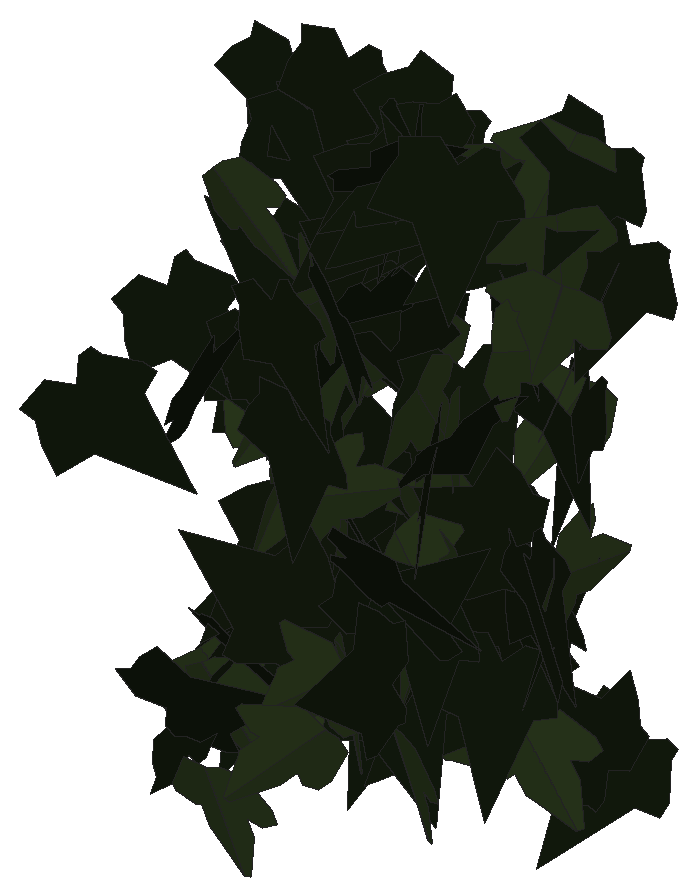
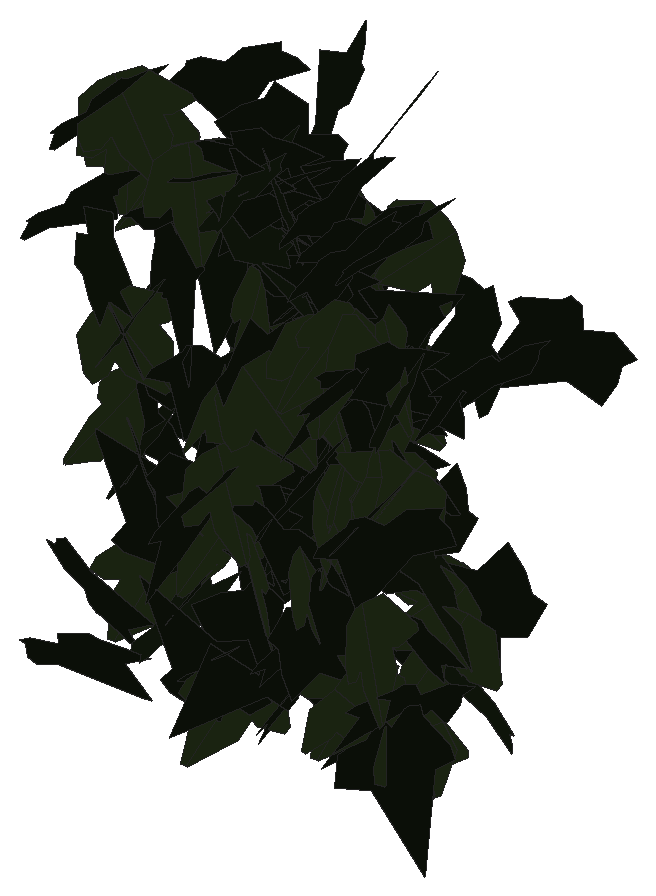
# SketchUp Ruby script. Lengths in inches.
U = 1.inch
M = Sketchup.active_model
def pt(a) = Geom::Point3d.new(a.map { |v| v * U })
def face(e, loops, mat)
  f = e.add_face(loops[0].map { |a| pt(a) })
  loops[1..].each { |l| e.add_face(l.map { |a| pt(a) }).erase! }
  f.material = f.back_material = mat if mat
  f
end
# faces: each face lists its corners as indices into pts; further lists are holes
def faces(e, pts, list, mat = nil) = list.each { |f| face(e, (f[0].is_a?(Array) ? f : [f]).map { |l| l.map { |i| pts[i] } }, mat) }
# xy, xz, yz: faces in a plane at the given z, y or x. An outline is a flat list of corners, or four numbers for a rectangle; further outlines are holes
def ring(l) = l.size == 4 ? [[l[0], l[1]], [l[2], l[1]], [l[2], l[3]], [l[0], l[3]]] : l.each_slice(2).to_a
def flat(e, list, mat, &to3) = list.each { |f| face(e, (f[0].is_a?(Array) ? f : [f]).map { |l| ring(l).map { |u, v| to3.(u, v) } }, mat) }
def xy(e, z, list, mat = nil) = flat(e, list, mat) { |x, y| [x, y, z] }
def xz(e, y, list, mat = nil) = flat(e, list, mat) { |x, z| [x, y, z] }
def yz(e, x, list, mat = nil) = flat(e, list, mat) { |y, z| [x, y, z] }
def lines(e, pts, list) = list.each { |a, b| e.add_line(pt(pts[a]), pt(pts[b])) }
# prism: a flat outline (further loops are holes) pulled along v
def prism(e, loops, v, mat = nil)
  f = face(e, loops, mat); d = Geom::Vector3d.new(v.map { |x| x * U })
  f.pushpull(f.normal.samedirection?(d) ? d.length : -d.length)
end
def box(e, o, s, mat = nil) = prism(e, [[o, [o[0] + s[0], o[1], o[2]], [o[0] + s[0], o[1] + s[1], o[2]], [o[0], o[1] + s[1], o[2]]]], [0, 0, s[2]], mat)
def at(x, y, z, deg = 0) = Geom::Transformation.translation(pt([x, y, z])) * Geom::Transformation.rotation(ORIGIN, Z_AXIS, deg.degrees)
def axes(o, x, y, z) = Geom::Transformation.new([*x, 0, *y, 0, *z, 0, *pt(o).to_a, 1])
def part(name) = M.definitions.add(name)
# library, detail: a bought-in or finely detailed component or shape, given as its bounding box
def library(name, o, s) = part(name).tap { |d| box(d.entities, o, s) }
def detail(e, o, s) = box(e.add_group.entities, o, s)
def put(e, d, t, mat = nil) = e.add_instance(d, t).tap { |i| i.material = mat if mat }
def group(e, t, mat = nil) = e.add_group.tap { |g| g.transformation = t; g.material = mat if mat }.entities
root = M.entities
M.materials.add("efeu1").color = [18, 25, 13]
M.materials.add("efeu2").color = [43, 57, 29]
c1 = part("ivyleaf_9")
p = [[1.54,2.16,1.25],[1.36,2.04,1.19],[-0.21,0.99,0.68],[-0.71,1.11,0.82],[-0.85,0.86,0.67],[-0.8,0.17,0.21],
  [-0.9,-0.01,0.1],[-0.67,-0.16,-0.02],[-0.08,-0.08,-0.05],[-0.03,-0.6,-0.4],[0.65,-0.88,-0.66],[0.83,-0.6,-0.49],
  [1.29,-0.42,-0.43],[1.8125,-0.07,-0.26],[1.21,0.44,0.15]]
faces(c1.entities,p,[[0,1,2,3,4,5,6,7,8,9,10,11,12,13,14]],"efeu1")
c2 = part("ivyleaf_10")
p = [[0,0.5,-0.03],[-0.0625,2.02,-0.43],[-0.19,2.01,-0.46],[-0.54,1.05,-0.29],[-0.52,0.625,-0.18],[-0.83,0.76,-0.28],
  [-1.16,0.64,-0.33],[-1.15,0.33,-0.24],[-0.77,-0.39,0.02],[-0.3,-0.51,0.16],[0.04,-0.48,0.23],[-0.02,2.01,-0.4375],
  [-0.06,2.01,-0.43],[0.04,-0.49,0.23],[0.67,-0.49,0.14],[1.38,0.36,-0.2],[1.375,0.51,-0.24],[0.81,0.65,-0.19],
  [0.62,0.59,-0.15],[0.6,1.09,-0.28],[0.5,1.23,-0.31]]
faces(c2.entities,p,[[0,1,2,3,4,5,6,7,8,9,10],[11,12,0,13,14,15,16,17,18,19,20]],"efeu2")
put(root,c1,axes([40.44,220.27,246.32],[0.16208,-0.38945,-0.26844],[0.03169,0.29207,-0.40459],[0.47194,0.11413,0.11936]))
put(root,c1,axes([40.98,221.25,242.32],[0.24181,0.19002,-0.39423],[-0.33477,-0.2098,-0.30646],[-0.28188,0.41216,0.02577]))
put(root,c1,axes([40.58,218.75,245.98],[-0.00232,-0.12946,-0.48294],[0.26446,0.40955,-0.11106],[0.42433,-0.25595,0.06657]))
put(root,c1,axes([40.75,221.67,244.9375],[-0.10521,-0.42408,-0.24307],[0.05609,0.23652,-0.43693],[0.48558,-0.11921,-0.0022]))
put(root,c1,axes([40.8,221.68,248.16],[-0.11399,-0.45265,0.17921],[0.02401,-0.18906,-0.46226],[0.48624,-0.09678,0.06484]))
put(root,c2,axes([40.99,220.93,242.1],[-0.09961,-0.48126,-0.09199],[0.00586,0.0927,-0.4913],[0.48994,-0.09896,-0.01282]))
put(root,c2,axes([41.04,221.55,243.63],[0.0308,-0.49854,-0.02258],[-0.00171,0.02252,-0.49949],[0.49905,0.03084,-0.00032]))
put(root,c1,axes([40.76,221.13,242.76],[0.14566,-0.34746,-0.32872],[0.08394,0.35686,-0.34001],[0.47089,0.04386,0.16229]))
put(root,c1,axes([41.27,219.52,242],[-0.37845,0.28286,-0.16361],[-0.1307,0.09841,0.47247],[0.29949,0.40038,-0.00055]))
put(root,c1,axes([40.91,221.3125,246.08],[0.02171,-0.27187,0.41907],[0.0689,-0.41382,-0.27204],[0.49475,0.06956,0.01949]))
put(root,c2,axes([41.41,220.84,246.49],[-0.27204,0.09807,0.40789],[-0.391,0.1169,-0.28889],[-0.15202,-0.47615,0.01309]))
put(root,c1,axes([41.27,221.42,246.47],[-0.33694,-0.35984,0.08358],[-0.06432,-0.05425,-0.49287],[0.36378,-0.34289,-0.00974]))
put(root,c2,axes([41.23,221.18,245.18],[0.04777,0.23287,-0.43987],[-0.10845,-0.42641,-0.23752],[-0.48575,0.1181,0.00977]))
put(root,c2,axes([40.98,221.0625,245.12],[0.36958,0.19046,0.27772],[0.22443,0.16812,-0.41396],[-0.25107,0.43065,0.03878]))
put(root,c1,axes([41,221.375,245.02],[0.26014,-0.39878,-0.15267],[-0.02205,0.16598,-0.47113],[0.42643,0.25185,0.06877]))
put(root,c2,axes([40.95,220.84,242.18],[-0.27106,-0.09475,-0.40933],[0.42005,-0.05039,-0.2665],[0.00925,-0.48835,0.10692]))
put(root,c2,axes([41.0625,220.44,247.59],[-0.34913,0.11494,-0.33897],[0.32423,-0.099,-0.36752],[-0.1516,-0.47643,-0.0054]))
put(root,c2,axes([41.33,221.57,242.76],[0.1825,0.34529,-0.3122],[-0.14436,-0.27682,-0.39055],[-0.44256,0.23268,-0.00135]))
put(root,c1,axes([41.35,219.25,245.77],[0.08753,0.14877,0.46926],[0.128,0.45335,-0.1676],[-0.47535,0.14947,0.04128]))
put(root,c1,axes([41.22,221.6875,247.97],[0.05816,-0.48707,-0.09686],[-0.01172,0.09615,-0.49053],[0.49647,0.05933,-0.00023]))
put(root,c2,axes([41.27,219.92,242.76],[-0.33136,-0.26762,-0.26188],[0.24862,0.10423,-0.4211],[0.27999,-0.40928,0.06399]))
put(root,c2,axes([41.3,221.33,242.82],[-0.38739,-0.23581,-0.21053],[0.23575,0.00633,-0.44089],[0.2106,-0.44086,0.10628]))
put(root,c1,axes([41.27,221.31,248.05],[-0.04877,-0.4417,-0.22918],[0.0279,0.22749,-0.44438],[0.49683,-0.05613,0.00246]))
put(root,c1,axes([41.8,220.65,246.45],[-0.00609,0.13398,0.48168],[-0.47214,0.15693,-0.04962],[-0.16447,-0.45544,0.1246]))
put(root,c1,axes([41.27,221.42,246.4],[0.19819,-0.38355,-0.25221],[-0.01826,0.26791,-0.42177],[0.45868,0.1764,0.09218]))
put(root,c1,axes([41.3125,220.55,246.05],[-0.18136,-0.21796,-0.41183],[0.33478,0.24642,-0.27785],[0.32409,-0.37652,0.05655]))
put(root,c1,axes([41.66,221.69,243.68],[-0.13173,0.22415,-0.42709],[0.17406,-0.39081,-0.25879],[-0.44984,-0.21686,0.02493]))
put(root,c1,axes([41.45,221.67,248.51],[0.00727,-0.49889,0.03256],[-0.01592,-0.03278,-0.49867],[0.49969,0.00622,-0.01636]))
put(root,c1,axes([41.89,219.7,243.48],[-0.25759,0.413,0.11435],[-0.07536,0.08768,-0.48645],[-0.42186,-0.26784,0.01707]))
put(root,c1,axes([41.22,219.3,242.54],[0.10449,-0.13173,0.47088],[0.45638,-0.14656,-0.14227],[0.1755,0.45953,0.08961]))
put(root,c1,axes([41.68,220.38,242.96],[-0.45556,-0.12577,-0.16324],[0.15565,0.04957,-0.47256],[0.13505,-0.48138,-0.00601]))
put(root,c2,axes([41.69,221.48,246.7],[-0.34193,-0.364,-0.02433],[0.01532,0.01898,-0.4994],[0.36449,-0.34226,-0.00183]))
put(root,c2,axes([41.59,221.29,246.75],[-0.09639,-0.32118,-0.37088],[0.19044,0.32384,-0.32994],[0.45215,-0.20487,0.0599]))
put(root,c2,axes([41.64,221.45,244.79],[0.12284,-0.42404,0.23474],[0.11413,-0.21004,-0.43915],[0.47105,0.16147,0.0452]))
put(root,c2,axes([41.78,221.57,244.06],[0.07186,-0.49282,0.04434],[-0.00324,-0.04528,-0.49794],[0.4948,0.07128,-0.0097]))
put(root,c2,axes([41.75,221.02,244.75],[0.10985,-0.41658,-0.25376],[0.05967,0.26964,-0.41681],[0.48412,0.06129,0.10896]))
put(root,c2,axes([41.64,219.52,242.85],[-0.41948,0.06518,-0.26417],[0.25554,-0.07237,-0.42363],[-0.09346,-0.49042,0.0274]))
put(root,c1,axes([41.52,220.88,245.39],[-0.13979,-0.11186,-0.46685],[0.44368,0.15558,-0.17013],[0.18333,-0.46182,0.05576]))
put(root,c1,axes([42.12,221.375,247.29],[-0.44983,-0.21695,0.02423],[-0.0134,-0.02796,-0.49904],[0.21789,-0.44961,0.01934]))
put(root,c2,axes([42.15,220.9,245.96],[-0.12388,-0.47377,0.10097],[0.00241,-0.10482,-0.48888],[0.4844,-0.12064,0.02825]))
put(root,c1,axes([41.92,221.36,243.24],[0.1556,-0.42092,-0.22049],[-0.02761,0.22361,-0.44636],[0.47437,0.15109,0.04634]))
put(root,c2,axes([42.34,221.72,246.01],[-0.26973,-0.3071,0.28798],[-0.19102,-0.21551,-0.40874],[0.37517,-0.33052,-0.00107]))
put(root,c1,axes([42.32,219.89,244.6],[-0.48355,-0.12698,-0.00729],[0.00658,0.00363,-0.49994],[0.12702,-0.48359,-0.00184]))
put(root,c2,axes([42.46,219.96,247.04],[-0.2431,0.12036,0.42002],[-0.40345,0.12267,-0.26867],[-0.16772,-0.46954,0.03748]))
put(root,c1,axes([42.04,221.65,244.44],[-0.29825,-0.19991,-0.34797],[0.3432,0.09763,-0.35026],[0.20799,-0.44778,0.07898]))
put(root,c1,axes([42.16,221.46,244.66],[-0.0575,-0.3964,0.29926],[-0.00934,-0.30034,-0.39963],[0.4966,-0.05155,0.02713]))
put(root,c1,axes([41.91,219.43,243.29],[0.1469,-0.27619,0.39005],[0.32512,-0.24135,-0.29334],[0.35031,0.33981,0.10868]))
put(root,c1,axes([42.26,221.01,246.83],[-0.18566,-0.31143,0.3443],[-0.02327,-0.3641,-0.34189],[0.46367,-0.14298,0.1207]))
put(root,c2,axes([42.33,218.61,242.38],[-0.49475,0.0394,-0.06056],[0.06045,-0.00383,-0.49632],[-0.03957,-0.49843,-0.00098]))
put(root,c2,axes([42.3,219.82,245.26],[-0.012,0.27146,-0.41972],[-0.01434,-0.41986,-0.27113],[-0.49965,0.00553,0.01786]))
put(root,c1,axes([42.15,221.16,242.53],[0.21146,-0.44611,-0.07917],[-0.02916,0.07379,-0.49367],[0.45214,0.2134,0.00519]))
put(root,c1,axes([42.625,220.99,247.81],[-0.3012,-0.33508,0.2168],[-0.15926,-0.14814,-0.45021],[0.36595,-0.34026,-0.01749]))
put(root,c1,axes([42.64,220.5,246.95],[-0.11834,0.39291,-0.28568],[0.07911,-0.27452,-0.41034],[-0.47931,-0.14232,0.00281]))
put(root,c1,axes([42.56,221.63,245.84],[-0.00384,-0.03793,0.49854],[-0.27489,-0.41629,-0.03379],[0.41764,-0.27435,-0.01766]))
put(root,c1,axes([42.41,221.37,248.26],[-0.26418,-0.00086,-0.42451],[0.41127,-0.12443,-0.25569],[-0.1052,-0.48427,0.06645]))
put(root,c1,axes([42.87,221.25,247.58],[-0.32351,0.38102,0.01303],[-0.06502,-0.03831,-0.49427],[-0.37566,-0.32149,0.07433]))
put(root,c1,axes([42.64,220.98,242.76],[-0.43786,-0.13681,-0.19891],[0.19256,0.05055,-0.45866],[0.14561,-0.47825,0.00842]))
put(root,c2,axes([42.64,220.36,243.51],[-0.34181,0.35785,0.0715],[-0.04332,0.05749,-0.49479],[-0.36234,-0.34444,-0.0083]))
put(root,c1,axes([42.77,221.49,248.53],[-0.44501,-0.22653,0.02555],[-0.01944,-0.01812,-0.49929],[0.22713,-0.44537,0.00732]))
put(root,c1,axes([42.43,221.36,242.98],[0.46637,0.17209,0.05369],[0.04903,0.0222,-0.49709],[-0.17347,0.46893,0.00383]))
put(root,c1,axes([42.67,220.87,243.65],[0.27045,-0.40309,0.1199],[-0.04156,0.11624,0.48452],[-0.41848,-0.27205,0.02937]))
put(root,c1,axes([42.79,221.3,247.87],[-0.33715,-0.29243,0.22543],[-0.05136,-0.26516,-0.42078],[0.36564,-0.30688,0.14876]))
put(root,c1,axes([42.64,220.6,248.29],[0.3319,0.3619,0.09417],[0.05805,0.07452,-0.491],[-0.36942,0.33686,0.00745]))
put(root,c1,axes([43.12,218.76,244.36],[-0.10997,0.17206,0.4564],[-0.45229,0.13917,-0.16144],[-0.18259,-0.44836,0.12503]))
put(root,c2,axes([42.88,221.15,243.65],[0.28172,-0.32908,-0.24968],[-0.15301,0.19758,-0.43307],[0.38369,0.32042,0.01062]))
put(root,c2,axes([42.61,219.82,245.11],[-0.07786,-0.08843,-0.48592],[0.27228,0.40273,-0.11692],[0.41207,-0.28282,-0.01456]))
put(root,c1,axes([42.57,221.66,248.11],[-0.00778,-0.38645,0.31717],[0.14645,-0.30505,-0.3681],[0.47801,0.08717,0.11793]))
put(root,c1,axes([43.09,221.23,248.28],[-0.47415,-0.08477,0.13414],[-0.10575,-0.1463,-0.46627],[0.1183,-0.47054,0.12081]))
put(root,c1,axes([42.67,219.43,246.02],[0.03892,-0.47276,0.15805],[0.02159,-0.15679,-0.47429],[0.49802,0.04374,0.00821]))
put(root,c1,axes([43.25,220.92,243.8125],[-0.34996,-0.03313,0.35557],[-0.35478,-0.02453,-0.35147],[0.04073,-0.4983,-0.00633]))
put(root,c1,axes([43.25,219.9,243.76],[-0.1896,0.01229,0.4625],[-0.45465,-0.09757,-0.18378],[0.08574,-0.49023,0.04817]))
put(root,c1,axes([43.25,219.85,243.17],[-0.00908,0.00988,0.49982],[-0.40507,0.29283,-0.01314],[-0.29298,-0.40516,0.00269]))
put(root,c1,axes([43.15,221.28,248.12],[-0.49084,-0.09467,-0.01088],[0.0104,0.00351,-0.49988],[0.09472,-0.49094,-0.00147]))
put(root,c2,axes([43.06,221.36,244.65],[-0.21097,-0.4433,0.09475],[-0.02826,-0.09144,-0.49075],[0.45243,-0.21242,0.01352]))
put(root,c2,axes([42.87,221.3125,242.27],[-0.26277,-0.32913,-0.26949],[0.2271,0.15929,-0.41599],[0.35969,-0.34103,0.06578]))
put(root,c1,axes([43.04,221.45,242.47],[-0.31424,-0.33366,0.19981],[-0.04742,-0.2221,-0.44545],[0.38601,-0.29891,0.10795]))
put(root,c1,axes([42.85,218.82,247.64],[0.2356,-0.43759,-0.05489],[-0.0199,0.05161,-0.49693],[0.44056,0.23634,0.0069]))
put(root,c1,axes([42.92,221.56,242.23],[-0.1764,0.1063,0.45561],[0.39368,-0.22936,0.20593],[0.25278,0.43139,-0.00278]))
put(root,c2,axes([43.28,221.6,248.16],[-0.2544,-0.42934,0.03079],[-0.01309,-0.02803,-0.49904],[0.43024,-0.25472,0.00302]))
put(root,c2,axes([43.2,221.27,245.52],[-0.06899,0.44621,-0.21478],[0.01086,-0.21544,-0.45107],[-0.4951,-0.06691,0.02004]))
put(root,c1,axes([43.125,221.59,244.43],[0.15993,-0.38066,-0.28199],[-0.11185,0.25887,-0.41289],[0.46034,0.19515,-0.00235]))
put(root,c2,axes([43.5,220.34,244.82],[-0.41806,0.1168,0.24816],[-0.23671,0.07484,-0.43401],[-0.13853,-0.48037,-0.00728]))
put(root,c1,axes([43.13,221.33,245.89],[-0.12027,-0.3928,-0.28504],[0.12707,0.25793,-0.40905],[0.46839,-0.17083,0.03778]))
put(root,c2,axes([43.14,221.09,244.01],[0.26809,0.30517,0.29155],[0.09834,0.29072,-0.39473],[-0.41043,0.26899,0.09585]))
put(root,c2,axes([43.27,219.36,243.67],[-0.29824,0.37708,-0.13735],[0.05878,-0.12823,-0.47969],[-0.39699,-0.30227,0.03215]))
put(root,c2,axes([43.38,220.35,246.17],[0.00055,-0.4089,-0.28776],[0.04959,0.28638,-0.40685],[0.49753,-0.02809,0.04087]))
put(root,c1,axes([43.6,221.1,244.39],[-0.14655,0.36243,-0.31172],[0.03473,-0.31711,-0.38502],[-0.47678,-0.1345,0.06777]))
put(root,c1,axes([43.26,220.09,243.21],[-0.20463,-0.27595,-0.36329],[0.21946,0.28952,-0.34353],[0.39995,-0.30005,0.00264]))
put(root,c1,axes([43.64,221.6,247.66],[-0.34156,-0.27858,0.23607],[-0.13553,-0.20344,-0.43617],[0.33907,-0.36194,0.06346]))
put(root,c1,axes([43.43,221.05,243.28],[0.13275,-0.47584,0.07716],[0.01957,-0.07465,-0.49401],[0.48166,0.13417,-0.00119]))
put(root,c1,axes([43.84,221.14,246.92],[0.21807,0.01013,-0.44983],[-0.44976,-0.00929,-0.21825],[-0.01278,0.49981,0.00506]))
put(root,c1,axes([44.12,220.74,244.68],[-0.23258,0.09197,0.43295],[-0.40263,0.15919,-0.2501],[-0.18384,-0.46497,0.00001]))
put(root,c1,axes([43.47,219.02,247.68],[0.12564,-0.30662,0.37443],[0.12079,-0.35474,-0.33102],[0.46864,0.17363,-0.01506]))
put(root,c2,axes([44.03,217.82,243.8125],[-0.21965,-0.25039,0.37291],[-0.25858,-0.26893,-0.33288],[0.36727,-0.33909,-0.01135]))
put(root,c2,axes([43.73,219.74,244.86],[-0.02624,0.47404,0.15685],[-0.00261,0.15693,-0.47473],[-0.4993,-0.02573,-0.00576]))
put(root,c2,axes([43.83,219.56,242.9],[-0.40495,0.2931,-0.0106],[0.00875,-0.00598,-0.49989],[-0.29316,-0.40504,-0.00029]))
put(root,c1,axes([43.74,220.46,248.7],[-0.18924,-0.44043,-0.14215],[0.07228,0.12356,-0.47907],[0.45713,-0.20187,0.0169]))
put(root,c1,axes([43.68,221.4,242.61],[-0.14549,-0.34562,0.33073],[0.14198,-0.36131,-0.31511],[0.45681,0.00223,0.20328]))
put(root,c2,axes([44.27,217.92,244.51],[-0.28528,-0.04572,0.40808],[-0.38957,-0.12697,-0.28656],[0.12983,-0.48144,0.03682]))
put(root,c2,axes([43.95,219.83,244.39],[0.11146,-0.42677,0.23546],[0.10655,-0.21437,-0.43897],[0.47563,0.14803,0.04316]))
put(root,c2,axes([44.22,221.54,248.61],[-0.371,-0.25664,0.21563],[-0.13111,-0.18491,-0.44567],[0.3085,-0.38722,0.06991]))
put(root,c1,axes([43.86,220.99,243.4375],[-0.14297,-0.0159,0.47886],[0.46421,-0.12833,0.13433],[0.11863,0.48299,0.05146]))
put(root,c1,axes([43.93,219.87,246.09],[-0.10668,-0.07508,-0.48268],[0.46142,-0.17767,-0.07435],[-0.16035,-0.4613,0.10719]))
put(root,c2,axes([44.32,221.49,245.98],[-0.25103,-0.32668,0.28331],[-0.07588,-0.28923,-0.40074],[0.42571,-0.24419,0.09563]))
put(root,c1,axes([44.34,219.64,246.39],[0.04368,0.49507,0.05479],[0.00483,0.05458,-0.49699],[-0.49807,0.04394,-0.00001]))
put(root,c1,axes([43.99,219.03,244.48],[-0.09354,-0.05887,0.48763],[0.48896,-0.05819,0.08677],[0.04654,0.4931,0.06845]))
put(root,c1,axes([44.13,219.54,244.58],[0.04277,-0.48722,0.10387],[0.01701,-0.10276,-0.48903],[0.49788,0.04536,0.00778]))
put(root,c1,axes([44.27,220.45,243.53],[-0.35916,-0.21372,-0.27446],[0.24266,0.12872,-0.41779],[0.24924,-0.43331,0.01127]))
put(root,c1,axes([44.47,221.72,246.99],[-0.29671,0.18965,-0.35496],[0.28286,-0.21543,-0.35154],[-0.28627,-0.40942,0.02055]))
put(root,c1,axes([44.18,221.37,246.07],[0.18396,-0.44926,0.11967],[0.0541,-0.10714,-0.48538],[0.46177,0.19153,0.00919]))
put(root,c1,axes([44.41,221.82,248.53],[-0.1576,-0.43938,0.17918],[-0.03025,-0.17912,-0.46583],[0.47355,-0.15768,0.02987]))
put(root,c2,axes([44.52,221.01,248.08],[-0.30003,-0.39814,-0.03822],[0.03521,0.0213,-0.4983],[0.39842,-0.30171,0.01525]))
put(root,c1,axes([44.44,220.94,244.12],[-0.33481,0.07188,-0.36433],[0.35064,-0.10035,-0.34203],[-0.12229,-0.48452,0.01679]))
put(root,c2,axes([44.48,220.65,242.75],[-0.41798,-0.18212,-0.20525],[0.22659,-0.01813,-0.44534],[0.15477,-0.4653,0.09769]))
put(root,c1,axes([44.55,221.4,246.13],[-0.35724,0.0375,-0.34782],[0.34406,-0.05227,-0.35901],[-0.06328,-0.49584,0.01154]))
put(root,c2,axes([44.54,220.1875,247.17],[0.06448,-0.20214,-0.45275],[0.14387,0.44455,-0.17799],[0.47449,-0.10732,0.11549]))
put(root,c1,axes([44.58,221.97,247.47],[-0.17844,-0.45254,0.11559],[0.0025,-0.12466,-0.4842],[0.46707,-0.17223,0.04675]))
put(root,c1,axes([44.74,221.83,242.26],[-0.43602,-0.24472,0.00002],[0.03288,-0.05862,-0.49546],[0.2425,-0.43206,0.06721]))
put(root,c1,axes([44.4,220.94,244.28],[0.12235,-0.4121,0.25535],[0.07563,-0.24391,-0.42987],[0.47886,0.14381,0.00265]))
put(root,c1,axes([44.29,218.21,245.66],[0.43984,-0.10355,0.21404],[0.20716,-0.05401,-0.45185],[0.1167,0.48617,-0.00461]))
put(root,c1,axes([45.04,221.07,242.48],[-0.09847,0.20513,0.44522],[-0.32448,0.31311,-0.21603],[-0.36744,-0.33148,0.07146]))
put(root,c1,axes([44.43,220.72,244.55],[-0.09661,-0.08783,-0.48265],[0.48284,0.07002,-0.10939],[0.08681,-0.48722,0.07128]))
put(root,c2,axes([44.91,220.52,247.66],[-0.43473,-0.18392,0.16487],[-0.13027,-0.11283,-0.46936],[0.20985,-0.45105,0.05018]))
put(root,c1,axes([44.77,218.14,244.54],[-0.07047,-0.13777,0.47545],[-0.21129,-0.42592,-0.15474],[0.44765,-0.22273,0.00181]))
put(root,c2,axes([44.76,220.81,244.6],[-0.03429,-0.13287,-0.4808],[0.09497,0.47138,-0.13704],[0.4897,-0.10072,-0.00709]))
